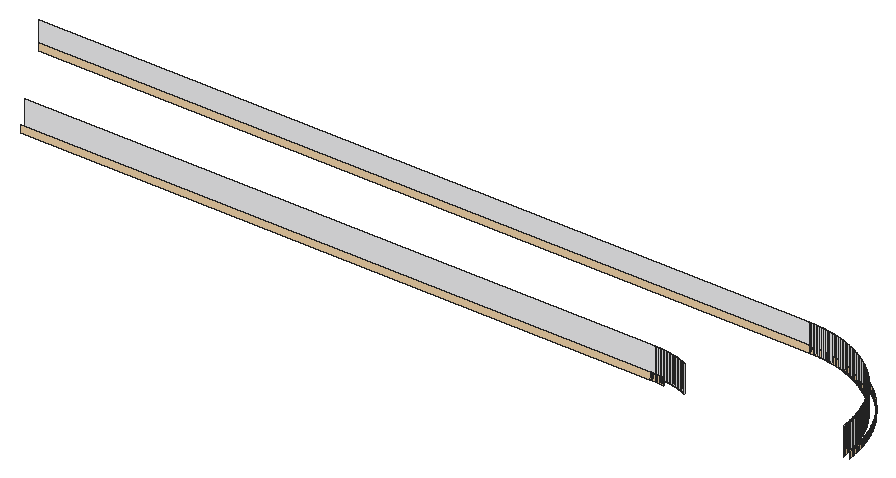
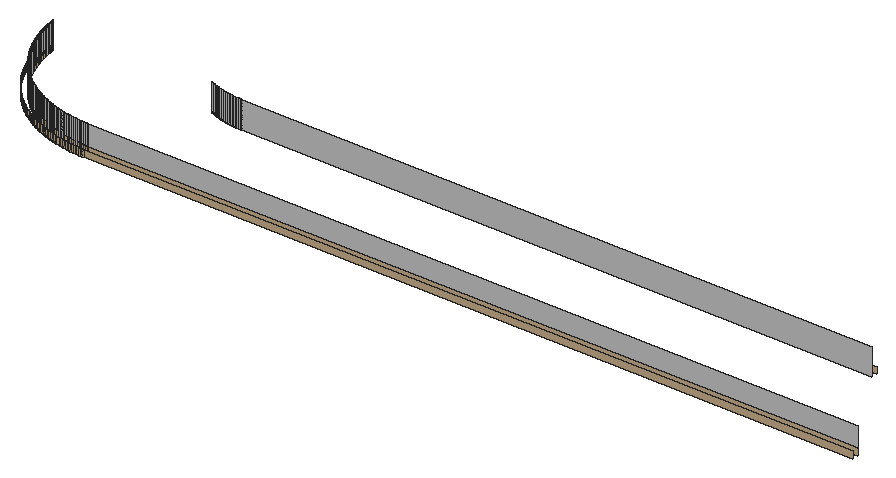
# SketchUp Ruby script. Lengths in inches.
U = 1.inch
M = Sketchup.active_model
def pt(a) = Geom::Point3d.new(a.map { |v| v * U })
def face(e, loops, mat)
  f = e.add_face(loops[0].map { |a| pt(a) })
  loops[1..].each { |l| e.add_face(l.map { |a| pt(a) }).erase! }
  f.material = f.back_material = mat if mat
  f
end
# faces: each face lists its corners as indices into pts; further lists are holes
def faces(e, pts, list, mat = nil) = list.each { |f| face(e, (f[0].is_a?(Array) ? f : [f]).map { |l| l.map { |i| pts[i] } }, mat) }
# xy, xz, yz: faces in a plane at the given z, y or x. An outline is a flat list of corners, or four numbers for a rectangle; further outlines are holes
def ring(l) = l.size == 4 ? [[l[0], l[1]], [l[2], l[1]], [l[2], l[3]], [l[0], l[3]]] : l.each_slice(2).to_a
def flat(e, list, mat, &to3) = list.each { |f| face(e, (f[0].is_a?(Array) ? f : [f]).map { |l| ring(l).map { |u, v| to3.(u, v) } }, mat) }
def xy(e, z, list, mat = nil) = flat(e, list, mat) { |x, y| [x, y, z] }
def xz(e, y, list, mat = nil) = flat(e, list, mat) { |x, z| [x, y, z] }
def yz(e, x, list, mat = nil) = flat(e, list, mat) { |y, z| [x, y, z] }
def lines(e, pts, list) = list.each { |a, b| e.add_line(pt(pts[a]), pt(pts[b])) }
# prism: a flat outline (further loops are holes) pulled along v
def prism(e, loops, v, mat = nil)
  f = face(e, loops, mat); d = Geom::Vector3d.new(v.map { |x| x * U })
  f.pushpull(f.normal.samedirection?(d) ? d.length : -d.length)
end
def box(e, o, s, mat = nil) = prism(e, [[o, [o[0] + s[0], o[1], o[2]], [o[0] + s[0], o[1] + s[1], o[2]], [o[0], o[1] + s[1], o[2]]]], [0, 0, s[2]], mat)
def at(x, y, z, deg = 0) = Geom::Transformation.translation(pt([x, y, z])) * Geom::Transformation.rotation(ORIGIN, Z_AXIS, deg.degrees)
def axes(o, x, y, z) = Geom::Transformation.new([*x, 0, *y, 0, *z, 0, *pt(o).to_a, 1])
def part(name) = M.definitions.add(name)
# library, detail: a bought-in or finely detailed component or shape, given as its bounding box
def library(name, o, s) = part(name).tap { |d| box(d.entities, o, s) }
def detail(e, o, s) = box(e.add_group.entities, o, s)
def put(e, d, t, mat = nil) = e.add_instance(d, t).tap { |i| i.material = mat if mat }
def group(e, t, mat = nil) = e.add_group.tap { |g| g.transformation = t; g.material = mat if mat }.entities
root = M.entities
M.materials.add("False Ceiling Light").color = [254, 223, 179]
M.materials.add("[Quartz Light Grey]").color = [251, 251, 252]
xz(root,218.5,[[56.99,115.32,165.01,116.49],[165.01,115.32,165.19,116.49],[165.19,115.32,165.38,116.49]],"False Ceiling Light")
xz(root,219.49,[[165.41,115.32,165.61,120]],"[Quartz Light Grey]")
xz(root,219.5,[[56.99,115.32,165.01,120],[165.01,115.32,165.2,120]],"[Quartz Light Grey]")
xz(root,237.5,[[45.01,115.32,176.99,116.49],[176.99,115.32,177.23,116.49],[177.23,115.32,177.45,116.49]],"False Ceiling Light")
xz(root,237.5,[[45.01,115.32,176.99,120],[176.99,115.32,177.23,120],[177.23,115.32,177.45,120]],"[Quartz Light Grey]")
xz(root,238.5,[[45,115.32,177,116.49],[177,115.32,177.24,116.49],[177.24,115.32,177.47,116.49]],"False Ceiling Light")
p = [[170.93,218.32,115.32],[171.12,218.24,115.32],[171.12,218.24,120],[170.93,218.32,120],[198.38,218.25,115.32],[198.36,218.47,115.32],
  [198.36,218.47,120],[198.38,218.25,120],[198.36,218.47,115.32],[198.38,218.25,115.32],[198.38,218.25,116.49],[198.36,218.47,116.49],
  [167.08,218.35,115.32],[166.89,218.375,115.32],[166.89,218.375,116.49],[167.08,218.35,116.49],[167.27,218.32,115.32],[167.27,218.32,116.49],
  [167.46,218.29,115.32],[167.46,218.29,116.49],[167.64,218.26,115.32],[167.64,218.26,116.49],[170.74,218.4,115.32],[170.74,218.4,120],
  [166.33,218.4375,115.32],[166.14,218.46,115.32],[166.14,218.46,116.49],[166.33,218.4375,116.49],[166.52,218.42,115.32],[166.52,218.42,116.49],
  [166.7,218.4,115.32],[166.7,218.4,116.49],[170.55,218.47,115.32],[170.55,218.47,120],[199.375,218.35,115.32],[199.35,218.59,115.32],
  [199.35,218.59,116.49],[199.375,218.35,116.49],[165.57,218.49,115.32],[165.38,218.5,115.32],[165.38,218.5,116.49],[165.57,218.49,116.49],
  [165.76,218.48,115.32],[165.76,218.48,116.49],[165.95,218.47,115.32],[165.95,218.47,116.49],[170.17,218.61,115.32],[170.36,218.54,115.32],
  [170.36,218.54,120],[170.17,218.61,120],[198.33,218.69,115.32],[198.33,218.69,120],[198.33,218.69,115.32],[198.33,218.69,116.49],
  [169.98,218.68,115.32],[169.98,218.68,120],[199.32,218.82,115.32],[199.32,218.82,116.49],[169.6,218.8,115.32],[169.79,218.74,115.32],
  [169.79,218.74,120],[169.6,218.8,120],[198.3,218.92,115.32],[198.3,218.92,120],[198.3,218.92,115.32],[198.3,218.92,116.49],
  [169.4,218.86,115.32],[169.4,218.86,120],[199.29,219.05,115.32],[199.29,219.05,116.49],[169.01,218.97,115.32],[169.21,218.92,115.32],
  [169.21,218.92,120],[169.01,218.97,120],[198.27,219.14,115.32],[198.27,219.14,120],[198.27,219.14,115.32],[198.27,219.14,116.49],
  [168.62,219.07,115.32],[168.82,219.02,115.32],[168.82,219.02,120],[168.62,219.07,120],[168.22,219.16,115.32],[168.42,219.12,115.32],
  [168.42,219.12,120],[168.22,219.16,120],[198.24,219.36,115.32],[198.24,219.36,120],[198.24,219.36,115.32],[198.24,219.36,116.49],
  [199.26,219.29,115.32],[199.26,219.29,116.49],[167.625,219.28,115.32],[167.82,219.24,115.32],[167.82,219.24,120],[167.625,219.28,120],
  [168.02,219.2,115.32],[168.02,219.2,120],[167.02,219.37,115.32],[167.22,219.34,115.32],[167.22,219.34,120],[167.02,219.37,120],
  [167.42,219.31,115.32],[167.42,219.31,120],[199.22,219.52,115.32],[199.22,219.52,116.49],[166.22,219.45,115.32],[166.42,219.44,115.32],
  [166.42,219.44,120],[166.22,219.45,120],[166.62,219.42,115.32],[166.62,219.42,120],[166.82,219.39,115.32],[166.82,219.39,120],
  [198.2,219.59,115.32],[198.2,219.59,120],[198.2,219.59,115.32],[198.2,219.59,116.49],[165.2,219.5,115.32],[165.41,219.49,115.32],
  [165.41,219.49,120],[165.2,219.5,120],[165.61,219.49,115.32],[165.8125,219.48,115.32],[165.8125,219.48,120],[165.61,219.49,120],
  [166.01,219.47,115.32],[166.01,219.47,120],[199.18,219.75,115.32],[199.18,219.75,116.49],[198.16,219.81,115.32],[198.16,219.81,120],
  [198.16,219.81,115.32],[198.16,219.81,116.49],[198.12,220.03,115.32],[198.12,220.03,120],[198.12,220.03,115.32],[198.12,220.03,116.49],
  [199.14,219.98,115.32],[199.14,219.98,116.49],[198.08,220.25,115.32],[198.08,220.25,120],[198.08,220.25,115.32],[198.08,220.25,116.49],
  [199.1,220.22,115.32],[199.1,220.22,116.49],[198.03,220.47,115.32],[198.03,220.47,120],[198.03,220.47,115.32],[198.03,220.47,116.49],
  [199.06,220.45,115.32],[199.06,220.45,116.49],[199.01,220.68,115.32],[199.01,220.68,116.49],[197.98,220.69,115.32],[197.98,220.69,120],
  [197.98,220.69,115.32],[197.98,220.69,116.49],[197.93,220.91,115.32],[197.93,220.91,120],[197.93,220.91,115.32],[197.93,220.91,116.49],
  [198.96,220.91,115.32],[198.96,220.91,116.49],[197.88,221.13,115.32],[197.88,221.13,120],[197.88,221.13,115.32],[197.88,221.13,116.49],
  [198.91,221.14,115.32],[198.91,221.14,116.49],[197.82,221.35,115.32],[197.82,221.35,120],[197.82,221.35,115.32],[197.82,221.35,116.49],
  [198.85,221.37,115.32],[198.85,221.37,116.49],[197.77,221.56,115.32],[197.77,221.56,120],[197.77,221.56,115.32],[197.77,221.56,116.49],
  [198.79,221.6,115.32],[198.79,221.6,116.49],[197.71,221.78,115.32],[197.71,221.78,120],[197.71,221.78,115.32],[197.71,221.78,116.49],
  [198.73,221.82,115.32],[198.73,221.82,116.49],[197.65,222,115.32],[197.65,222,120],[197.65,222,115.32],[197.65,222,116.49],
  [198.67,222.05,115.32],[198.67,222.05,116.49],[197.58,222.21,115.32],[197.58,222.21,120],[197.58,222.21,115.32],[197.58,222.21,116.49],
  [198.61,222.28,115.32],[198.61,222.28,116.49],[197.52,222.43,115.32],[197.52,222.43,120],[197.52,222.43,115.32],[197.52,222.43,116.49],
  [198.54,222.5,115.32],[198.54,222.5,116.49],[197.45,222.64,115.32],[197.45,222.64,120],[197.45,222.64,115.32],[197.45,222.64,116.49],
  [198.47,222.73,115.32],[198.47,222.73,116.49],[197.375,222.86,115.32],[197.375,222.86,120],[197.375,222.86,115.32],[197.375,222.86,116.49],
  [198.4,222.95,115.32],[198.4,222.95,116.49],[197.3,223.07,115.32],[197.3,223.07,120],[197.3,223.07,115.32],[197.3,223.07,116.49],
  [198.32,223.18,115.32],[198.32,223.18,116.49],[197.23,223.28,115.32],[197.23,223.28,120],[197.23,223.28,115.32],[197.23,223.28,116.49],
  [198.25,223.4,115.32],[198.25,223.4,116.49],[197.15,223.49,115.32],[197.15,223.49,120],[197.15,223.49,115.32],[197.15,223.49,116.49],
  [198.17,223.62,115.32],[198.17,223.62,116.49],[197.07,223.7,115.32],[197.07,223.7,120],[197.07,223.7,115.32],[197.07,223.7,116.49],
  [198.09,223.84,115.32],[198.09,223.84,116.49],[196.99,223.91,115.32],[196.99,223.91,120],[196.99,223.91,115.32],[196.99,223.91,116.49],
  [198.01,224.0625,115.32],[198.01,224.0625,116.49],[196.91,224.125,115.32],[196.91,224.125,120],[196.91,224.125,115.32],[196.91,224.125,116.49],
  [196.82,224.33,115.32],[196.82,224.33,120],[196.82,224.33,115.32],[196.82,224.33,116.49],[197.92,224.28,115.32],[197.92,224.28,116.49],
  [196.73,224.54,115.32],[196.73,224.54,120],[196.73,224.54,115.32],[196.73,224.54,116.49],[197.83,224.5,115.32],[197.83,224.5,116.49],
  [196.64,224.74,115.32],[196.64,224.74,120],[196.64,224.74,115.32],[196.64,224.74,116.49],[197.74,224.72,115.32],[197.74,224.72,116.49],
  [196.55,224.95,115.32],[196.55,224.95,120],[196.55,224.95,115.32],[196.55,224.95,116.49],[197.65,224.9375,115.32],[197.65,224.9375,116.49],
  [197.55,225.15,115.32],[197.55,225.15,116.49],[196.45,225.15,115.32],[196.45,225.15,120],[196.45,225.15,115.32],[196.45,225.15,116.49],
  [196.36,225.36,115.32],[196.36,225.36,120],[196.36,225.36,115.32],[196.36,225.36,116.49],[197.46,225.37,115.32],[197.46,225.37,116.49],
  [196.26,225.56,115.32],[196.26,225.56,120],[196.26,225.56,115.32],[196.26,225.56,116.49],[197.36,225.58,115.32],[197.36,225.58,116.49],
  [196.16,225.76,115.32],[196.16,225.76,120],[196.16,225.76,115.32],[196.16,225.76,116.49],[197.26,225.79,115.32],[197.26,225.79,116.49],
  [196.05,225.96,115.32],[196.05,225.96,120],[196.05,225.96,115.32],[196.05,225.96,116.49],[197.15,226,115.32],[197.15,226,116.49],
  [195.95,226.16,115.32],[195.95,226.16,120],[195.95,226.16,115.32],[195.95,226.16,116.49],[197.05,226.21,115.32],[197.05,226.21,116.49],
  [195.84,226.36,115.32],[195.84,226.36,120],[195.84,226.36,115.32],[195.84,226.36,116.49],[196.94,226.42,115.32],[196.94,226.42,116.49],
  [195.73,226.55,115.32],[195.73,226.55,120],[195.73,226.55,115.32],[195.73,226.55,116.49],[196.83,226.63,115.32],[196.83,226.63,116.49],
  [195.62,226.75,115.32],[195.62,226.75,120],[195.62,226.75,115.32],[195.62,226.75,116.49],[196.72,226.84,115.32],[196.72,226.84,116.49],
  [195.51,226.94,115.32],[195.51,226.94,120],[195.51,226.94,115.32],[195.51,226.94,116.49],[196.6,227.05,115.32],[196.6,227.05,116.49],
  [195.39,227.14,115.32],[195.39,227.14,120],[195.39,227.14,115.32],[195.39,227.14,116.49],[196.49,227.25,115.32],[196.49,227.25,116.49],
  [195.27,227.33,115.32],[195.27,227.33,120],[195.27,227.33,115.32],[195.27,227.33,116.49],[196.37,227.45,115.32],[196.37,227.45,116.49],
  [195.15,227.52,115.32],[195.15,227.52,120],[195.15,227.52,115.32],[195.15,227.52,116.49],[195.03,227.71,115.32],[195.03,227.71,120],
  [195.03,227.71,115.32],[195.03,227.71,116.49],[196.25,227.66,115.32],[196.25,227.66,116.49],[194.91,227.9,115.32],[194.91,227.9,120],
  [194.91,227.9,115.32],[194.91,227.9,116.49],[196.12,227.86,115.32],[196.12,227.86,116.49],[194.78,228.08,115.32],[194.78,228.08,120],
  [194.78,228.08,115.32],[194.78,228.08,116.49],[196,228.06,115.32],[196,228.06,116.49],[194.65,228.27,115.32],[194.65,228.27,120],
  [194.65,228.27,115.32],[194.65,228.27,116.49],[195.87,228.25,115.32],[195.87,228.25,116.49],[194.53,228.45,115.32],[194.53,228.45,120],
  [194.53,228.45,115.32],[194.53,228.45,116.49],[195.74,228.45,115.32],[195.74,228.45,116.49],[194.39,228.64,115.32],[194.39,228.64,120],
  [194.39,228.64,115.32],[194.39,228.64,116.49],[195.61,228.65,115.32],[195.61,228.65,116.49],[194.26,228.82,115.32],[194.26,228.82,120],
  [194.26,228.82,115.32],[194.26,228.82,116.49],[195.48,228.84,115.32],[195.48,228.84,116.49],[194.125,229,115.32],[194.125,229,120],
  [194.125,229,115.32],[194.125,229,116.49],[195.34,229.03,115.32],[195.34,229.03,116.49],[193.99,229.18,115.32],[193.99,229.18,120],
  [193.99,229.18,115.32],[193.99,229.18,116.49],[195.2,229.23,115.32],[195.2,229.23,116.49],[193.85,229.35,115.32],[193.85,229.35,120],
  [193.85,229.35,115.32],[193.85,229.35,116.49],[195.0625,229.42,115.32],[195.0625,229.42,116.49],[193.71,229.53,115.32],[193.71,229.53,120],
  [193.71,229.53,115.32],[193.71,229.53,116.49],[194.92,229.6,115.32],[194.92,229.6,116.49],[193.57,229.7,115.32],[193.57,229.7,120],
  [193.57,229.7,115.32],[193.57,229.7,116.49],[194.78,229.79,115.32],[194.78,229.79,116.49],[193.42,229.88,115.32],[193.42,229.88,120],
  [193.42,229.88,115.32],[193.42,229.88,116.49],[194.63,229.98,115.32],[194.63,229.98,116.49],[193.28,230.05,115.32],[193.28,230.05,120],
  [193.28,230.05,115.32],[193.28,230.05,116.49],[193.13,230.22,115.32],[193.13,230.22,120],[193.13,230.22,115.32],[193.13,230.22,116.49],
  [194.49,230.16,115.32],[194.49,230.16,116.49],[192.98,230.39,115.32],[192.98,230.39,120],[192.98,230.39,115.32],[192.98,230.39,116.49],
  [194.34,230.34,115.32],[194.34,230.34,116.49],[194.19,230.52,115.32],[194.19,230.52,116.49],[192.83,230.55,115.32],[192.83,230.55,120],
  [192.83,230.55,115.32],[192.83,230.55,116.49],[194.03,230.7,115.32],[194.03,230.7,116.49],[192.67,230.72,115.32],[192.67,230.72,120],
  [192.67,230.72,115.32],[192.67,230.72,116.49],[192.52,230.88,115.32],[192.52,230.88,120],[192.52,230.88,115.32],[192.52,230.88,116.49],
  [193.88,230.88,115.32],[193.88,230.88,116.49],[192.36,231.04,115.32],[192.36,231.04,120],[192.36,231.04,115.32],[192.36,231.04,116.49],
  [193.72,231.06,115.32],[193.72,231.06,116.49],[192.2,231.2,115.32],[192.2,231.2,120],[192.2,231.2,115.32],[192.2,231.2,116.49],
  [193.5625,231.23,115.32],[193.5625,231.23,116.49],[192.04,231.36,115.32],[192.04,231.36,120],[192.04,231.36,115.32],[192.04,231.36,116.49],
  [193.4,231.4,115.32],[193.4,231.4,116.49],[191.88,231.52,115.32],[191.88,231.52,120],[191.88,231.52,115.32],[191.88,231.52,116.49],
  [193.24,231.57,115.32],[193.24,231.57,116.49],[191.72,231.67,115.32],[191.72,231.67,120],[191.72,231.67,115.32],[191.72,231.67,116.49],
  [193.08,231.74,115.32],[193.08,231.74,116.49],[191.55,231.83,115.32],[191.55,231.83,120],[191.55,231.83,115.32],[191.55,231.83,116.49],
  [192.91,231.91,115.32],[192.91,231.91,116.49],[191.39,231.98,115.32],[191.39,231.98,120],[191.39,231.98,115.32],[191.39,231.98,116.49],
  [192.74,232.08,115.32],[192.74,232.08,116.49],[191.22,232.13,115.32],[191.22,232.13,120],[191.22,232.13,115.32],[191.22,232.13,116.49],
  [191.05,232.28,115.32],[191.05,232.28,120],[191.05,232.28,115.32],[191.05,232.28,116.49],[192.57,232.24,115.32],[192.57,232.24,116.49],
  [192.4,232.4,115.32],[192.4,232.4,116.49],[190.88,232.42,115.32],[190.88,232.42,120],[190.88,232.42,115.32],[190.88,232.42,116.49],
  [190.7,232.57,115.32],[190.7,232.57,120],[190.7,232.57,115.32],[190.7,232.57,116.49],[192.23,232.5625,115.32],[192.23,232.5625,116.49],
  [190.53,232.71,115.32],[190.53,232.71,120],[190.53,232.71,115.32],[190.53,232.71,116.49],[192.06,232.72,115.32],[192.06,232.72,116.49],
  [190.35,232.85,115.32],[190.35,232.85,120],[190.35,232.85,115.32],[190.35,232.85,116.49],[191.88,232.88,115.32],[191.88,232.88,116.49],
  [190.18,232.99,115.32],[190.18,232.99,120],[190.18,232.99,115.32],[190.18,232.99,116.49],[191.7,233.03,115.32],[191.7,233.03,116.49],
  [190,233.125,115.32],[190,233.125,120],[190,233.125,115.32],[190,233.125,116.49],[191.52,233.19,115.32],[191.52,233.19,116.49],
  [189.82,233.26,115.32],[189.82,233.26,120],[189.82,233.26,115.32],[189.82,233.26,116.49],[191.34,233.34,115.32],[191.34,233.34,116.49],
  [189.64,233.39,115.32],[189.64,233.39,120],[189.64,233.39,115.32],[189.64,233.39,116.49],[191.16,233.49,115.32],[191.16,233.49,116.49],
  [189.45,233.53,115.32],[189.45,233.53,120],[189.45,233.53,115.32],[189.45,233.53,116.49],[189.27,233.65,115.32],[189.27,233.65,120],
  [189.27,233.65,115.32],[189.27,233.65,116.49],[190.98,233.63,115.32],[190.98,233.63,116.49],[190.79,233.78,115.32],[190.79,233.78,116.49],
  [189.08,233.78,115.32],[189.08,233.78,120],[189.08,233.78,115.32],[189.08,233.78,116.49],[188.9,233.91,115.32],[188.9,233.91,120],
  [188.9,233.91,115.32],[188.9,233.91,116.49],[190.6,233.92,115.32],[190.6,233.92,116.49],[188.71,234.03,115.32],[188.71,234.03,120],
  [188.71,234.03,115.32],[188.71,234.03,116.49],[190.42,234.0625,115.32],[190.42,234.0625,116.49],[188.52,234.15,115.32],[188.52,234.15,120],
  [188.52,234.15,115.32],[188.52,234.15,116.49],[190.23,234.2,115.32],[190.23,234.2,116.49],[188.33,234.27,115.32],[188.33,234.27,120],
  [188.33,234.27,115.32],[188.33,234.27,116.49],[190.03,234.34,115.32],[190.03,234.34,116.49],[188.14,234.39,115.32],[188.14,234.39,120],
  [188.14,234.39,115.32],[188.14,234.39,116.49],[189.84,234.48,115.32],[189.84,234.48,116.49],[187.94,234.51,115.32],[187.94,234.51,120],
  [187.94,234.51,115.32],[187.94,234.51,116.49],[187.75,234.62,115.32],[187.75,234.62,120],[187.75,234.62,115.32],[187.75,234.62,116.49],
  [189.65,234.61,115.32],[189.65,234.61,116.49],[187.55,234.73,115.32],[187.55,234.73,120],[187.55,234.73,115.32],[187.55,234.73,116.49],
  [189.45,234.74,115.32],[189.45,234.74,116.49],[187.36,234.84,115.32],[187.36,234.84,120],[187.36,234.84,115.32],[187.36,234.84,116.49],
  [189.25,234.87,115.32],[189.25,234.87,116.49],[187.16,234.95,115.32],[187.16,234.95,120],[187.16,234.95,115.32],[187.16,234.95,116.49],
  [186.96,235.05,115.32],[186.96,235.05,120],[186.96,235.05,115.32],[186.96,235.05,116.49],[189.06,235,115.32],[189.06,235,116.49],
  [188.86,235.12,115.32],[188.86,235.12,116.49],[186.76,235.16,115.32],[186.76,235.16,120],[186.76,235.16,115.32],[186.76,235.16,116.49],
  [188.66,235.25,115.32],[188.66,235.25,116.49],[186.56,235.26,115.32],[186.56,235.26,120],[186.56,235.26,115.32],[186.56,235.26,116.49],
  [188.45,235.37,115.32],[188.45,235.37,116.49],[186.36,235.36,115.32],[186.36,235.36,120],[186.36,235.36,115.32],[186.36,235.36,116.49],
  [186.15,235.45,115.32],[186.15,235.45,120],[186.15,235.45,115.32],[186.15,235.45,116.49],[188.25,235.49,115.32],[188.25,235.49,116.49],
  [185.95,235.55,115.32],[185.74,235.64,115.32],[185.74,235.64,120],[185.95,235.55,120],[185.74,235.64,115.32],[185.95,235.55,115.32],
  [185.95,235.55,116.49],[185.74,235.64,116.49],[188.05,235.6,115.32],[188.05,235.6,116.49],[185.54,235.73,115.32],[185.54,235.73,120],
  [185.54,235.73,115.32],[185.54,235.73,116.49],[187.84,235.72,115.32],[187.84,235.72,116.49],[185.33,235.82,115.32],[185.33,235.82,120],
  [185.33,235.82,115.32],[185.33,235.82,116.49],[187.63,235.83,115.32],[187.63,235.83,116.49],[185.125,235.91,115.32],[185.125,235.91,120],
  [185.125,235.91,115.32],[185.125,235.91,116.49],[187.42,235.94,115.32],[187.42,235.94,116.49],[184.91,235.99,115.32],[184.91,235.99,120],
  [184.91,235.99,115.32],[184.91,235.99,116.49],[187.21,236.05,115.32],[187.21,236.05,116.49],[184.7,236.07,115.32],[184.7,236.07,120],
  [184.7,236.07,115.32],[184.7,236.07,116.49],[187,236.15,115.32],[187,236.15,116.49],[184.49,236.15,115.32],[184.49,236.15,120],
  [184.49,236.15,115.32],[184.49,236.15,116.49],[184.28,236.23,115.32],[184.07,236.3,115.32],[184.07,236.3,120],[184.28,236.23,120],
  [184.07,236.3,115.32],[184.28,236.23,115.32],[184.28,236.23,116.49],[184.07,236.3,116.49],[186.79,236.26,115.32],[186.79,236.26,116.49],
  [183.86,236.375,115.32],[183.86,236.375,120],[183.86,236.375,115.32],[183.86,236.375,116.49],[186.58,236.36,115.32],[186.58,236.36,116.49],
  [183.64,236.45,115.32],[183.43,236.52,115.32],[183.43,236.52,120],[183.64,236.45,120],[183.43,236.52,115.32],[183.64,236.45,115.32],
  [183.64,236.45,116.49],[183.43,236.52,116.49],[186.37,236.46,115.32],[186.37,236.46,116.49],[183.21,236.58,115.32],[183.21,236.58,120],
  [183.21,236.58,115.32],[183.21,236.58,116.49],[186.15,236.55,115.32],[186.15,236.55,116.49],[183,236.65,115.32],[182.78,236.71,115.32],
  [182.78,236.71,120],[183,236.65,120],[182.78,236.71,115.32],[183,236.65,115.32],[183,236.65,116.49],[182.78,236.71,116.49],
  [185.9375,236.65,115.32],[185.72,236.74,115.32],[185.72,236.74,116.49],[185.9375,236.65,116.49],[182.56,236.77,115.32],[182.56,236.77,120],
  [182.56,236.77,115.32],[182.56,236.77,116.49],[185.5,236.83,115.32],[185.5,236.83,116.49],[182.35,236.82,115.32],[182.13,236.88,115.32],
  [182.13,236.88,120],[182.35,236.82,120],[182.13,236.88,115.32],[182.35,236.82,115.32],[182.35,236.82,116.49],[182.13,236.88,116.49],
  [185.28,236.92,115.32],[185.28,236.92,116.49],[181.91,236.93,115.32],[181.69,236.98,115.32],[181.69,236.98,120],[181.91,236.93,120],
  [181.69,236.98,115.32],[181.91,236.93,115.32],[181.91,236.93,116.49],[181.69,236.98,116.49],[185.0625,237.01,115.32],[185.0625,237.01,116.49],
  [181.47,237.03,115.32],[181.25,237.08,115.32],[181.25,237.08,120],[181.47,237.03,120],[181.25,237.08,115.32],[181.47,237.03,115.32],
  [181.47,237.03,116.49],[181.25,237.08,116.49],[184.84,237.09,115.32],[184.84,237.09,116.49],[181.03,237.12,115.32],[180.81,237.16,115.32],
  [180.81,237.16,120],[181.03,237.12,120],[180.81,237.16,115.32],[181.03,237.12,115.32],[181.03,237.12,116.49],[180.81,237.16,116.49],
  [184.62,237.17,115.32],[184.62,237.17,116.49],[180.36,237.24,115.32],[180.14,237.27,115.32],[180.14,237.27,120],[180.36,237.24,120],
  [180.14,237.27,115.32],[180.36,237.24,115.32],[180.36,237.24,116.49],[180.14,237.27,116.49],[180.59,237.2,115.32],[180.59,237.2,120],
  [180.59,237.2,115.32],[180.59,237.2,116.49],[184.4,237.25,115.32],[184.18,237.32,115.32],[184.18,237.32,116.49],[184.4,237.25,116.49],
  [179.69,237.33,115.32],[179.47,237.36,115.32],[179.47,237.36,120],[179.69,237.33,120],[179.47,237.36,115.32],[179.69,237.33,115.32],
  [179.69,237.33,116.49],[179.47,237.36,116.49],[179.92,237.3,115.32],[179.92,237.3,120],[179.92,237.3,115.32],[179.92,237.3,116.49],
  [183.95,237.4,115.32],[183.95,237.4,116.49],[178.57,237.44,115.32],[178.35,237.46,115.32],[178.35,237.46,120],[178.57,237.44,120],
  [178.35,237.46,115.32],[178.57,237.44,115.32],[178.57,237.44,116.49],[178.35,237.46,116.49],[178.8,237.42,115.32],[178.8,237.42,120],
  [178.8,237.42,115.32],[178.8,237.42,116.49],[179.02,237.4,115.32],[179.02,237.4,120],[179.02,237.4,115.32],[179.02,237.4,116.49],
  [179.25,237.38,115.32],[179.25,237.38,120],[179.25,237.38,115.32],[179.25,237.38,116.49],[183.73,237.47,115.32],[183.73,237.47,116.49],
  [177.68,237.49,115.32],[177.45,237.5,115.32],[177.45,237.5,120],[177.68,237.49,120],[177.45,237.5,115.32],[177.68,237.49,115.32],
  [177.68,237.49,116.49],[177.45,237.5,116.49],[177.9,237.48,115.32],[177.9,237.48,120],[177.9,237.48,115.32],[177.9,237.48,116.49],
  [178.125,237.47,115.32],[178.125,237.47,120],[178.125,237.47,115.32],[178.125,237.47,116.49],[183.5,237.54,115.32],[183.28,237.61,115.32],
  [183.28,237.61,116.49],[183.5,237.54,116.49],[183.05,237.67,115.32],[183.05,237.67,116.49],[182.82,237.73,115.32],[182.6,237.79,115.32],
  [182.6,237.79,116.49],[182.82,237.73,116.49],[182.37,237.85,115.32],[182.37,237.85,116.49],[182.14,237.91,115.32],[181.91,237.96,115.32],
  [181.91,237.96,116.49],[182.14,237.91,116.49],[181.68,238.01,115.32],[181.45,238.06,115.32],[181.45,238.06,116.49],[181.68,238.01,116.49],
  [180.98,238.14,115.32],[180.75,238.18,115.32],[180.75,238.18,116.49],[180.98,238.14,116.49],[181.22,238.1,115.32],[181.22,238.1,116.49],
  [180.52,238.22,115.32],[180.29,238.26,115.32],[180.29,238.26,116.49],[180.52,238.22,116.49],[179.82,238.32,115.32],[179.59,238.35,115.32],
  [179.59,238.35,116.49],[179.82,238.32,116.49],[180.05,238.29,115.32],[180.05,238.29,116.49],[178.65,238.44,115.32],[178.41,238.46,115.32],
  [178.41,238.46,116.49],[178.65,238.44,116.49],[178.88,238.42,115.32],[178.88,238.42,116.49],[179.12,238.4,115.32],[179.12,238.4,116.49],
  [179.35,238.375,115.32],[179.35,238.375,116.49],[177.71,238.49,115.32],[177.47,238.5,115.32],[177.47,238.5,116.49],[177.71,238.49,116.49],
  [177.94,238.48,115.32],[177.94,238.48,116.49],[178.18,238.47,115.32],[178.18,238.47,116.49]]
faces(root,p,[[0,1,2,3],[4,5,6,7],[22,0,3,23],[32,22,23,33],[46,47,48,49],[47,32,33,48],[5,50,51,6],[54,46,49,55],
  [58,59,60,61],[59,54,55,60],[50,62,63,51],[66,58,61,67],[70,71,72,73],[71,66,67,72],[62,74,75,63],[78,79,80,81],
  [79,70,73,80],[82,83,84,85],[83,78,81,84],[74,86,87,75],[92,93,94,95],[93,96,97,94],[96,82,85,97],[98,99,100,101],
  [99,102,103,100],[102,92,95,103],[106,107,108,109],[107,110,111,108],[110,112,113,111],[112,98,101,113],[86,114,115,87],[118,119,120,121],
  [122,123,124,125],[123,126,127,124],[126,106,109,127],[114,130,131,115],[130,134,135,131],[134,140,141,135],[140,146,147,141],[146,154,155,147],
  [154,158,159,155],[158,164,165,159],[164,170,171,165],[170,176,177,171],[176,182,183,177],[182,188,189,183],[188,194,195,189],[194,200,201,195],
  [200,206,207,201],[206,212,213,207],[212,218,219,213],[218,224,225,219],[224,230,231,225],[230,236,237,231],[236,242,243,237],[242,248,249,243],
  [248,252,253,249],[252,258,259,253],[258,264,265,259],[264,270,271,265],[270,278,279,271],[278,282,283,279],[282,288,289,283],[288,294,295,289],
  [294,300,301,295],[300,306,307,301],[306,312,313,307],[312,318,319,313],[318,324,325,319],[324,330,331,325],[330,336,337,331],[336,342,343,337],
  [342,348,349,343],[348,352,353,349],[352,358,359,353],[358,364,365,359],[364,370,371,365],[370,376,377,371],[376,382,383,377],[382,388,389,383],
  [388,394,395,389],[394,400,401,395],[400,406,407,401],[406,412,413,407],[412,418,419,413],[418,424,425,419],[424,430,431,425],[430,434,435,431],
  [434,440,441,435],[440,448,449,441],[448,454,455,449],[454,458,459,455],[458,464,465,459],[464,470,471,465],[470,476,477,471],[476,482,483,477],
  [482,488,489,483],[488,494,495,489],[494,500,501,495],[500,506,507,501],[506,510,511,507],[510,518,519,511],[518,522,523,519],[522,528,529,523],
  [528,534,535,529],[534,540,541,535],[540,546,547,541],[546,552,553,547],[552,558,559,553],[558,564,565,559],[564,568,569,565],[568,576,577,569],
  [576,580,581,577],[580,586,587,581],[586,592,593,587],[592,598,599,593],[598,604,605,599],[604,610,611,605],[610,614,615,611],[614,620,621,615],
  [620,626,627,621],[626,632,633,627],[632,636,637,633],[636,644,645,637],[644,650,651,645],[650,656,657,651],[656,660,661,657],[666,667,668,669],
  [660,666,669,661],[667,676,677,668],[676,682,683,677],[682,688,689,683],[688,694,695,689],[694,700,701,695],[700,706,707,701],[710,711,712,713],
  [706,710,713,707],[711,720,721,712],[726,727,728,729],[720,726,729,721],[727,736,737,728],[742,743,744,745],[736,742,745,737],[743,754,755,744],
  [760,761,762,763],[754,760,763,755],[770,771,772,773],[761,770,773,762],[780,781,782,783],[771,780,783,772],[790,791,792,793],[781,790,793,782],
  [800,801,802,803],[808,800,803,809],[791,808,809,792],[816,817,818,819],[824,816,819,825],[801,824,825,802],[830,831,832,833],[838,830,833,839],
  [842,838,839,843],[846,842,843,847],[817,846,847,818],[852,853,854,855],[860,852,855,861],[864,860,861,865],[831,864,865,832]],"[Quartz Light Grey]")
faces(root,p,[[8,9,10,11],[12,13,14,15],[16,12,15,17],[18,16,17,19],[20,18,19,21],[24,25,26,27],[28,24,27,29],[30,28,29,31],
  [13,30,31,14],[34,35,36,37],[38,39,40,41],[42,38,41,43],[44,42,43,45],[25,44,45,26],[52,8,11,53],[35,56,57,36],
  [64,52,53,65],[56,68,69,57],[76,64,65,77],[88,76,77,89],[68,90,91,69],[90,104,105,91],[116,88,89,117],[104,128,129,105],
  [132,116,117,133],[136,132,133,137],[128,138,139,129],[142,136,137,143],[138,144,145,139],[148,142,143,149],[144,150,151,145],[150,152,153,151],
  [156,148,149,157],[160,156,157,161],[152,162,163,153],[166,160,161,167],[162,168,169,163],[172,166,167,173],[168,174,175,169],[178,172,173,179],
  [174,180,181,175],[184,178,179,185],[180,186,187,181],[190,184,185,191],[186,192,193,187],[196,190,191,197],[192,198,199,193],[202,196,197,203],
  [198,204,205,199],[208,202,203,209],[204,210,211,205],[214,208,209,215],[210,216,217,211],[220,214,215,221],[216,222,223,217],[226,220,221,227],
  [222,228,229,223],[232,226,227,233],[228,234,235,229],[238,232,233,239],[234,240,241,235],[244,238,239,245],[240,246,247,241],[250,244,245,251],
  [254,250,251,255],[246,256,257,247],[260,254,255,261],[256,262,263,257],[266,260,261,267],[262,268,269,263],[272,266,267,273],[268,274,275,269],
  [274,276,277,275],[280,272,273,281],[284,280,281,285],[276,286,287,277],[290,284,285,291],[286,292,293,287],[296,290,291,297],[292,298,299,293],
  [302,296,297,303],[298,304,305,299],[308,302,303,309],[304,310,311,305],[314,308,309,315],[310,316,317,311],[320,314,315,321],[316,322,323,317],
  [326,320,321,327],[322,328,329,323],[332,326,327,333],[328,334,335,329],[338,332,333,339],[334,340,341,335],[344,338,339,345],[340,346,347,341],
  [350,344,345,351],[354,350,351,355],[346,356,357,347],[360,354,355,361],[356,362,363,357],[366,360,361,367],[362,368,369,363],[372,366,367,373],
  [368,374,375,369],[378,372,373,379],[374,380,381,375],[384,378,379,385],[380,386,387,381],[390,384,385,391],[386,392,393,387],[396,390,391,397],
  [392,398,399,393],[402,396,397,403],[398,404,405,399],[408,402,403,409],[404,410,411,405],[414,408,409,415],[410,416,417,411],[420,414,415,421],
  [416,422,423,417],[426,420,421,427],[422,428,429,423],[432,426,427,433],[436,432,433,437],[428,438,439,429],[442,436,437,443],[438,444,445,439],
  [444,446,447,445],[450,442,443,451],[446,452,453,447],[456,450,451,457],[460,456,457,461],[452,462,463,453],[466,460,461,467],[462,468,469,463],
  [472,466,467,473],[468,474,475,469],[478,472,473,479],[474,480,481,475],[484,478,479,485],[480,486,487,481],[490,484,485,491],[486,492,493,487],
  [496,490,491,497],[492,498,499,493],[502,496,497,503],[498,504,505,499],[508,502,503,509],[512,508,509,513],[504,514,515,505],[514,516,517,515],
  [520,512,513,521],[524,520,521,525],[516,526,527,517],[530,524,525,531],[526,532,533,527],[536,530,531,537],[532,538,539,533],[542,536,537,543],
  [538,544,545,539],[548,542,543,549],[544,550,551,545],[554,548,549,555],[550,556,557,551],[560,554,555,561],[556,562,563,557],[566,560,561,567],
  [570,566,567,571],[562,572,573,563],[572,574,575,573],[578,570,571,579],[582,578,579,583],[574,584,585,575],[588,582,583,589],[584,590,591,585],
  [594,588,589,595],[590,596,597,591],[600,594,595,601],[596,602,603,597],[606,600,601,607],[602,608,609,603],[612,606,607,613],[616,612,613,617],
  [608,618,619,609],[622,616,617,623],[618,624,625,619],[628,622,623,629],[624,630,631,625],[634,628,629,635],[638,634,635,639],[630,640,641,631],
  [640,642,643,641],[646,638,639,647],[642,648,649,643],[652,646,647,653],[648,654,655,649],[658,652,653,659],[662,658,659,663],[654,664,665,655],
  [670,671,672,673],[671,662,663,672],[664,674,675,665],[678,670,673,679],[674,680,681,675],[684,678,679,685],[680,686,687,681],[690,684,685,691],
  [686,692,693,687],[696,690,691,697],[692,698,699,693],[702,696,697,703],[698,704,705,699],[708,702,703,709],[714,715,716,717],[715,708,709,716],
  [704,718,719,705],[722,714,717,723],[718,724,725,719],[730,731,732,733],[731,722,723,732],[724,734,735,725],[738,730,733,739],[734,740,741,735],
  [746,747,748,749],[747,738,739,748],[750,751,752,753],[740,750,753,741],[756,746,749,757],[751,758,759,752],[764,765,766,767],[765,756,757,766],
  [758,768,769,759],[774,775,776,777],[775,764,767,776],[768,778,779,769],[784,785,786,787],[785,774,777,786],[778,788,789,779],[794,795,796,797],
  [795,784,787,796],[788,798,799,789],[804,805,806,807],[805,810,811,806],[810,794,797,811],[812,813,814,815],[798,812,815,799],[820,821,822,823],
  [821,826,827,822],[826,804,807,827],[813,828,829,814],[834,835,836,837],[835,840,841,836],[840,844,845,841],[844,848,849,845],[848,820,823,849],
  [828,850,851,829],[856,857,858,859],[857,862,863,858],[862,866,867,863],[866,834,837,867],[868,869,870,871],[850,868,871,851],[869,872,873,870],
  [874,875,876,877],[872,874,877,873],[875,878,879,876],[880,881,882,883],[878,880,883,879],[884,885,886,887],[881,884,887,882],[888,889,890,891],
  [892,888,891,893],[885,892,893,886],[894,895,896,897],[889,894,897,890],[898,899,900,901],[902,898,901,903],[895,902,903,896],[904,905,906,907],
  [908,904,907,909],[910,908,909,911],[912,910,911,913],[899,912,913,900],[914,915,916,917],[918,914,917,919],[920,918,919,921],[905,920,921,906]],"False Ceiling Light")
